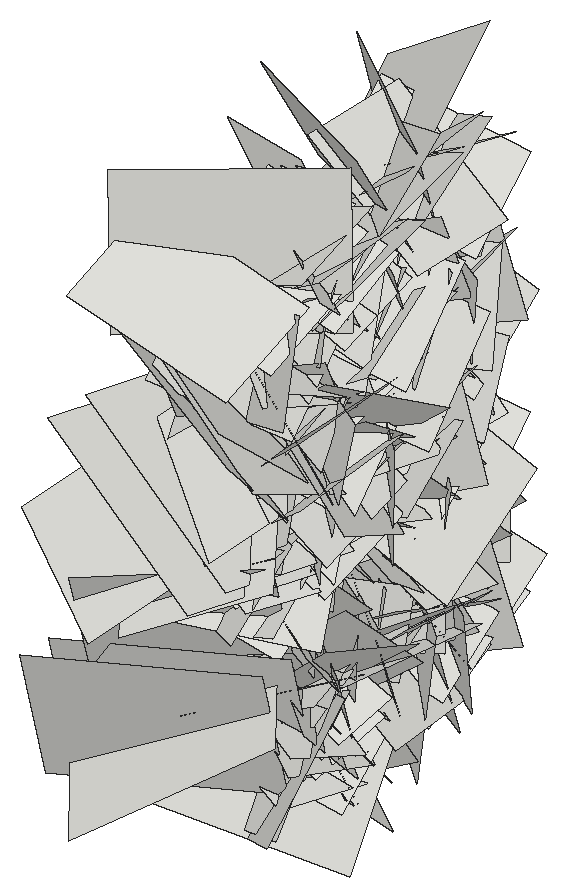
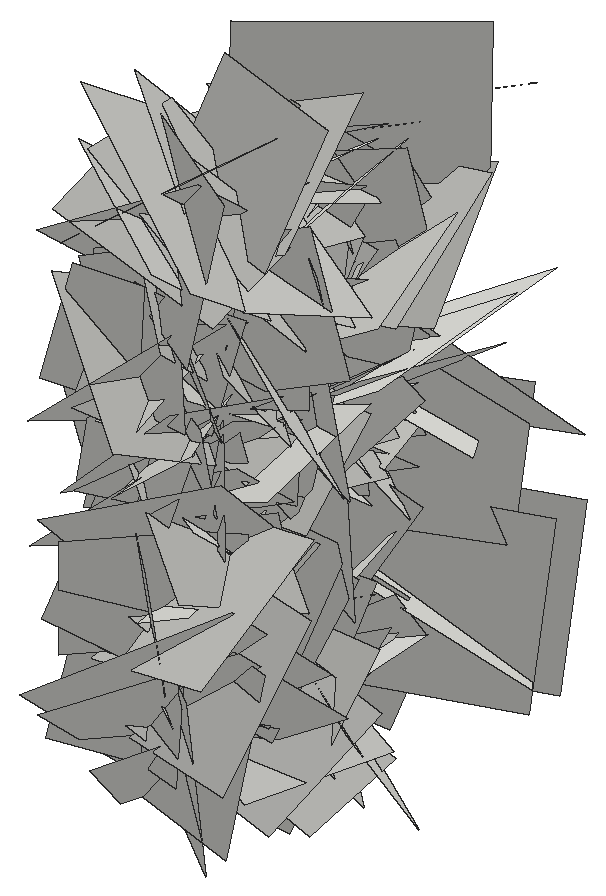
# SketchUp Ruby script. Lengths in inches.
U = 1.inch
M = Sketchup.active_model
def pt(a) = Geom::Point3d.new(a.map { |v| v * U })
def face(e, loops, mat)
  f = e.add_face(loops[0].map { |a| pt(a) })
  loops[1..].each { |l| e.add_face(l.map { |a| pt(a) }).erase! }
  f.material = f.back_material = mat if mat
  f
end
# faces: each face lists its corners as indices into pts; further lists are holes
def faces(e, pts, list, mat = nil) = list.each { |f| face(e, (f[0].is_a?(Array) ? f : [f]).map { |l| l.map { |i| pts[i] } }, mat) }
# xy, xz, yz: faces in a plane at the given z, y or x. An outline is a flat list of corners, or four numbers for a rectangle; further outlines are holes
def ring(l) = l.size == 4 ? [[l[0], l[1]], [l[2], l[1]], [l[2], l[3]], [l[0], l[3]]] : l.each_slice(2).to_a
def flat(e, list, mat, &to3) = list.each { |f| face(e, (f[0].is_a?(Array) ? f : [f]).map { |l| ring(l).map { |u, v| to3.(u, v) } }, mat) }
def xy(e, z, list, mat = nil) = flat(e, list, mat) { |x, y| [x, y, z] }
def xz(e, y, list, mat = nil) = flat(e, list, mat) { |x, z| [x, y, z] }
def yz(e, x, list, mat = nil) = flat(e, list, mat) { |y, z| [x, y, z] }
def lines(e, pts, list) = list.each { |a, b| e.add_line(pt(pts[a]), pt(pts[b])) }
# prism: a flat outline (further loops are holes) pulled along v
def prism(e, loops, v, mat = nil)
  f = face(e, loops, mat); d = Geom::Vector3d.new(v.map { |x| x * U })
  f.pushpull(f.normal.samedirection?(d) ? d.length : -d.length)
end
def box(e, o, s, mat = nil) = prism(e, [[o, [o[0] + s[0], o[1], o[2]], [o[0] + s[0], o[1] + s[1], o[2]], [o[0], o[1] + s[1], o[2]]]], [0, 0, s[2]], mat)
def at(x, y, z, deg = 0) = Geom::Transformation.translation(pt([x, y, z])) * Geom::Transformation.rotation(ORIGIN, Z_AXIS, deg.degrees)
def axes(o, x, y, z) = Geom::Transformation.new([*x, 0, *y, 0, *z, 0, *pt(o).to_a, 1])
def part(name) = M.definitions.add(name)
# library, detail: a bought-in or finely detailed component or shape, given as its bounding box
def library(name, o, s) = part(name).tap { |d| box(d.entities, o, s) }
def detail(e, o, s) = box(e.add_group.entities, o, s)
def put(e, d, t, mat = nil) = e.add_instance(d, t).tap { |i| i.material = mat if mat }
def group(e, t, mat = nil) = e.add_group.tap { |g| g.transformation = t; g.material = mat if mat }.entities
root = M.entities
c1 = part("Component\#6")
p = [[0.01,0,0],[0,3.24,4.54],[4.32,3.24,4.54],[4.33,0,0]]
faces(c1.entities,p,[[0,1,2,3]])
put(root,c1,axes([18.61,125.5,13.2],[-1.07209,0.56535,0.5401],[-0.40295,0.41611,-1.14744],[-0.72423,-1.06841,-0.1611]))
put(root,c1,axes([18.5,125.3125,7.6875],[-0.15543,0.49215,-1.26812],[-0.29157,-1.25984,-0.45713],[-1.41209,0.20597,0.23397]))
put(root,c1,axes([18.5,126.76,7.6875],[-0.15543,0.49215,-1.26812],[-0.29157,-1.25984,-0.45713],[-1.41209,0.20597,0.23397]))
put(root,c1,axes([18.5,135.96,3.29],[-0.1622,-0.76384,1.11136],[-0.23079,1.11781,0.7383],[-1.4107,-0.09505,-0.24857]))
put(root,c1,axes([18.5,130.15,15.41],[-0.24379,0.89731,1.03665],[-0.02149,1.04879,-0.91232],[-1.45316,-0.16605,-0.16042]))
put(root,c1,axes([18.5,136.82,5.83],[-0.1656,-1.02965,0.80161],[-0.14776,0.81588,1.02082],[-1.37528,0.03632,-0.2062]))
put(root,c1,axes([18.5,130.78,10.54],[-0.24762,-1.26357,-0.1726],[0.00687,-0.17664,1.28442],[-1.3518,0.23056,0.03815]))
put(root,c1,axes([19.67,124.5,5.79],[-0.83668,1.07369,0.2523],[-0.21003,0.16716,-1.33127],[-1.15009,-0.81162,0.05958]))
put(root,c1,axes([18.5,138.98,4.78],[-0.22268,-0.9196,-0.8307],[-0.07298,-0.83259,0.9391],[-1.31157,0.20246,0.08879]))
put(root,c1,axes([18.5,129.98,10.23],[-0.10909,-1.3698,0.20566],[0.00727,0.20572,1.37363],[-1.46824,0.1028,-0.00848]))
put(root,c1,axes([18.5,128.0625,10.23],[-0.10909,-1.3698,0.20566],[0.00727,0.20572,1.37363],[-1.46824,0.1028,-0.00848]))
put(root,c1,axes([18.5,135.39,1.18],[-0.01455,-0.40823,1.27358],[-0.1801,1.26386,0.40328],[-1.40617,-0.15765,-0.06483]))
put(root,c1,axes([18.5,137,19.49],[-0.23927,-0.1296,-1.18474],[-0.04055,-1.20439,0.13904],[-1.26266,0.06324,0.22004]))
put(root,c1,axes([18.5,127.67,13.74],[-0.06329,-0.97705,0.81505],[-0.12838,0.8166,0.97005],[-1.34259,-0.03203,-0.13118]))
put(root,c1,axes([18.5,125.99,1.35],[-0.00241,0.79041,1.08039],[-0.06651,1.07914,-0.78963],[-1.41741,-0.05198,0.03522]))
put(root,c1,axes([18.5,132.12,7.08],[0.00585,1.22451,-0.43101],[-0.11167,-0.42917,-1.22063],[-1.3715,0.04016,0.09755]))
put(root,c1,axes([18.5,133.15,22.79],[-0.15509,1.06813,0.73269],[0.10614,0.74447,-1.06531],[-1.36888,-0.06329,-0.16562]))
put(root,c1,axes([18.5,128.24,17.68],[-0.22785,0.52614,1.07761],[0.06777,1.09826,-0.52347],[-1.26934,-0.03581,-0.22138]))
put(root,c1,axes([18.5,133.04,19.75],[-0.14526,-0.49923,0.95494],[-0.24012,0.95446,0.46647],[-1.11669,-0.1403,-0.22453]))
put(root,c1,axes([18.5,139.8125,5.82],[-0.12038,-0.94885,-0.86303],[0.08352,-0.86993,0.94607],[-1.35702,0.03063,0.13479]))
put(root,c1,axes([18.5,131.95,0.87],[-0.07095,-0.70744,0.83659],[-0.30432,0.82019,0.6706],[-1.12076,-0.17792,-0.23504]))
put(root,c1,axes([18.5,125.82,11.42],[-0.20547,0.4933,-0.99975],[-0.03886,-1.01702,-0.49472],[-1.18108,-0.05236,0.1902]))
put(root,c1,axes([18.5,129.66,12.47],[0.1081,-1.2535,0.58167],[0.00417,0.58351,1.25678],[-1.46479,-0.09085,0.0465]))
put(root,c1,axes([18.5,129.48,20.64],[0.14207,1.22324,0.51937],[-0.11373,0.53026,-1.2212],[-1.40407,0.08082,0.15147]))
put(root,c1,axes([18.5,134.94,17.85],[-0.08672,-0.29938,1.1859],[0.04442,1.18717,0.30259],[-1.29573,0.06074,-0.069]))
put(root,c1,axes([18.5,133.96,9.66],[-0.06967,-1.04066,0.34132],[-0.1454,0.34706,1.03175],[-1.15177,0.01914,-0.15089]))
put(root,c1,axes([18.5,126.61,12.8],[0.1414,-0.87971,0.87765],[-0.19082,0.8597,0.88908],[-1.30331,-0.22132,-0.03495]))
put(root,c1,axes([18.5,129.42,5.47],[0.26825,1.30607,0.06413],[-0.25565,0.11082,-1.30519],[-1.36232,0.23638,0.25756]))
put(root,c1,axes([18.5,136.29,19.65],[-0.239,0.33681,-1.04778],[0.13934,-1.05364,-0.36698],[-1.15826,-0.19625,0.17205]))
put(root,c1,axes([18.5,131.16,1.32],[-0.11103,-1.00768,0.14491],[-0.13016,0.15712,1.00381],[-1.07125,0.08535,-0.13699]))
put(root,c1,axes([18.5,129.81,24.32],[0.08615,-0.07511,-1.33483],[0.12267,-1.33188,0.08199],[-1.41184,-0.12031,-0.07433]))
put(root,c1,axes([14.53,129.35,18.22],[-0.07955,-0.40219,0.442],[-0.06566,0.44831,0.39741],[0.63004,-0.00406,0.09723]))
put(root,c1,axes([18.5,130,20.12],[0.02742,-1.01137,-0.35231],[-0.21232,-0.35076,0.99222],[-1.1152,0.04191,-0.19757]))
put(root,c1,axes([18.5,127.69,20.12],[0.02742,-1.01137,-0.35231],[-0.21232,-0.35076,0.99222],[-1.1152,0.04191,-0.19757]))
put(root,c1,axes([14.53,138.1,17.99],[-0.00934,-0.49027,-0.41508],[-0.1892,-0.3969,0.47259],[0.65411,-0.1218,0.13076]))
put(root,c1,axes([18.5,127.92,6.47],[0.03611,0.05394,1.13531],[-0.09971,1.13206,-0.05096],[-1.20066,-0.09239,0.03838]))
put(root,c1,axes([19.22,124.93,11.12],[-0.54058,0.75668,0.32998],[-0.30141,0.20311,-0.90522],[-0.82148,-0.57246,0.11499]))
put(root,c1,axes([18.5,134.14,22.88],[-0.03825,0.99518,-0.25742],[-0.13842,-0.25993,-0.98657],[-1.08078,-0.00193,0.13547]))
put(root,c1,axes([14.53,134.77,2.57],[-0.05447,0.40704,0.46107],[-0.08155,0.45478,-0.41007],[0.64681,0.09162,-0.01288]))
put(root,c1,axes([18.5,131.18,15.16],[-0.15294,-1.16278,0.39158],[0.28955,0.35393,1.15166],[-1.26792,0.22109,0.21577]))
put(root,c1,axes([18.5,131.94,16.85],[0.08825,-0.96476,0.81898],[0.08011,0.82307,0.9619],[-1.33903,-0.01434,0.11152]))
put(root,c1,axes([18.5,128.56,10.3125],[0.23413,0.04823,1.24691],[-0.1221,1.26168,-0.02839],[-1.31707,-0.10839,0.22429]))
put(root,c1,axes([18.5,133.91,11.1875],[0.02059,0.92356,-0.8814],[0.20413,-0.87353,-0.91107],[-1.33776,-0.11908,-0.15259]))
put(root,c1,axes([18.5,130.99,8.6],[-0.04494,-0.64922,0.68663],[-0.20873,0.6783,0.62918],[-0.97967,-0.11474,-0.16555]))
put(root,c1,axes([18.5,129.625,19.87],[0.14331,0.9196,0.97349],[0.15794,0.96203,-0.92947],[-1.41069,0.20113,-0.00516]))
put(root,c1,axes([18.5,137.87,11.82],[-0.23548,-0.98581,-0.19043],[0.17104,-0.22756,0.98976],[-1.05044,0.18394,0.20385]))
put(root,c1,axes([14.53,131.8,8.64],[-0.08497,0.05507,0.67491],[-0.04101,0.67814,-0.05993],[0.71661,0.04534,0.0766]))
put(root,c1,axes([18.5,134.95,12.42],[-0.03363,0.92541,-1.00089],[0.39451,-0.95725,-0.89685],[-1.39004,-0.29406,-0.23032]))
put(root,c1,axes([14.53,131.9,7.66],[-0.03371,0.19161,0.61883],[-0.06203,0.6162,-0.1938],[0.68388,0.06533,0.01292]))
put(root,c1,axes([18.5,131.74,20.5625],[0.11289,-0.41624,-1.03402],[-0.06809,-1.03929,0.41174],[-1.17957,0.02016,-0.12272]))
put(root,c1,axes([18.5,138.97,11.375],[0.02639,-0.72989,-0.72722],[-0.07911,-0.7268,0.72691],[-1.08928,0.0351,-0.07041]))
put(root,c1,axes([18.5,128.87,2.92],[-0.01411,0.95221,-0.19006],[-0.11482,-0.19035,-0.94606],[-1.02282,0.00823,0.10882]))
put(root,c1,axes([14.53,134.26,15.51],[-0.13639,0.72841,-0.25059],[-0.07067,-0.26364,-0.7321],[0.81346,0.09922,-0.10562]))
put(root,c1,axes([18.5,129.68,16.21],[-0.16446,-0.17941,-0.82447],[-0.07006,-0.83314,0.19373],[-0.89165,0.09856,0.13685]))
put(root,c1,axes([14.53,127.28,0.51],[-0.04452,-0.40985,0.5808],[-0.07759,0.58122,0.40485],[0.7495,0.03582,0.07641]))
put(root,c1,axes([18.5,133.2,0.29],[0.16868,0.00753,1.30134],[0.16064,1.302,-0.02607],[-1.37005,0.15359,0.15716]))
put(root,c1,axes([14.53,134.57,7.51],[-0.06425,-0.0713,-0.65597],[0.02618,-0.65852,0.06929],[0.69893,0.01811,-0.0629]))
put(root,c1,axes([18.5,128.52,17.74],[-0.08604,0.43028,-0.81229],[-0.04293,-0.81633,-0.42838],[-0.97342,-0.00203,0.0907]))
put(root,c1,axes([14.53,132.11,13.83],[-0.12823,-0.67114,-0.46171],[-0.10246,-0.45164,0.68184],[0.85739,-0.15435,0.01243]))
put(root,c1,axes([18.5,133.79,15.82],[-0.11741,-0.82822,-0.37202],[-0.00882,-0.37384,0.83474],[-0.96237,0.10447,0.03774]))
put(root,c1,axes([14.53,131.53,3.64],[-0.03356,0.34972,-0.55611],[0.01458,-0.55628,-0.35061],[0.69619,0.02851,-0.01946]))
put(root,c1,axes([14.53,130.57,14.69],[-0.08088,0.56373,-0.36339],[0.06437,-0.35843,-0.56878],[0.70803,0.09698,0.0102]))
put(root,c1,axes([18.5,130.125,12.36],[0.14413,1.23778,0.56401],[0.30073,0.52855,-1.22835],[-1.41013,0.23923,-0.20431]))
put(root,c1,axes([18.5,129.28,18.375],[-0.15104,-0.37703,-0.77667],[0.00911,-0.78776,0.38083],[-0.9151,0.05438,0.13199]))
put(root,c1,axes([18.5,132.6,22.9],[-0.05818,0.99288,0.05669],[0.07779,0.06066,-0.99145],[-1.05129,-0.05046,-0.07649]))
put(root,c1,axes([14.53,133.3125,17.59],[0.01529,0.27468,0.5349],[0.08187,0.52978,-0.27413],[0.6321,-0.07526,0.02257]))
put(root,c1,axes([14.53,129.84,16.13],[0.05288,0.68465,0.04631],[-0.09068,0.05228,-0.68068],[0.72171,-0.04359,-0.08892]))
put(root,c1,axes([18.5,129.45,15.69],[0.00555,0.72683,0.86308],[0.19522,0.85097,-0.71774],[-1.18002,0.1442,-0.11468]))
put(root,c1,axes([14.53,129.41,10.95],[-0.18775,-0.48629,-0.69123],[0.00245,-0.70652,0.49646],[0.89586,-0.09998,-0.14623]))
put(root,c1,axes([14.53,132.63,6.14],[-0.10731,0.87556,-0.00554],[-0.12201,-0.01884,-0.87366],[0.92006,0.09962,-0.1165]))
put(root,c1,axes([18.5,133.96,12.5],[-0.03937,0.24323,0.81298],[-0.12274,0.80469,-0.24604],[-0.89109,-0.12158,-0.00203]))
put(root,c1,axes([18.5,127.6,6.32],[-0.09105,0.77875,-0.27248],[-0.08108,-0.28029,-0.77696],[-0.87078,-0.05533,0.10084]))
put(root,c1,axes([18.5,133.1,9.3125],[0.02086,0.87239,-0.16813],[-0.14049,-0.16341,-0.8634],[-0.93122,0.04419,0.12649]))
put(root,c1,axes([18.5,131.05,1.96],[0.03915,-1.05631,0.36623],[0.17317,0.36759,1.04378],[-1.17236,0.01903,0.16641]))
put(root,c1,axes([14.53,133.88,6.93],[-0.12434,-0.60409,0.41763],[0.12699,0.40152,0.61444],[0.76804,-0.16419,-0.03398]))
put(root,c1,axes([18.5,136.93,7.59],[0.11136,0.24127,-0.97313],[-0.07388,-0.97433,-0.24909],[-1.06018,0.09324,-0.08486]))
put(root,c1,axes([14.53,130.03,2.94],[-0.11679,-0.3481,0.76621],[-0.04914,0.77408,0.34502],[0.89071,-0.00294,0.1195]))
put(root,c1,axes([14.53,129.23,5.41],[-0.17398,-0.60139,0.60701],[0.02487,0.6147,0.61536],[0.9054,-0.13245,0.09973]))
put(root,c1,axes([18.5,132.5,3.06],[0.12033,-0.77552,-0.96336],[0.26418,-0.93322,0.78062],[-1.28404,-0.26468,0.07033]))
put(root,c1,axes([14.53,129.18,10.77],[0.08644,0.04023,-0.60323],[0.06997,-0.60565,-0.03147],[0.63702,0.06107,0.08531]))
put(root,c1,axes([18.5,132.55,10.48],[0.11298,-1.07137,-0.22101],[0.09706,-0.21254,1.07447],[-1.1555,-0.12261,0.06864]))
put(root,c1,axes([14.53,128.34,18.92],[0.04874,0.38349,0.62334],[-0.06251,0.62448,-0.37984],[0.77325,0.02631,-0.07]))
put(root,c1,axes([14.53,129.8,15.91],[0.05085,-0.71724,0.33006],[-0.13843,0.31891,0.71198],[0.82538,0.09767,0.09907]))
put(root,c1,axes([18.5,127.86,19.19],[0.25173,1.01088,0.57921],[0.04385,0.58343,-1.03521],[-1.23418,0.22691,0.08136]))
put(root,c1,axes([18.5,127.34,21.1],[0.03089,0.79811,0.32897],[-0.11706,0.3299,-0.79059],[-0.90753,-0.01539,0.11317]))
put(root,c1,axes([14.53,133.42,16.97],[-0.14677,0.94615,0.46149],[-0.22557,0.4307,-0.94687],[1.09283,0.21597,-0.13346]))
put(root,c1,axes([14.53,133.96,6.46],[-0.0893,0.11056,0.97068],[-0.19494,0.95507,-0.12474],[1.01706,0.19277,0.06132]))
put(root,c1,axes([18.5,136.53,11.26],[0.01536,-0.64622,-0.54667],[-0.11065,-0.54394,0.64022],[-0.89037,0.05645,-0.089]))
put(root,c1,axes([14.53,131.99,-0.9375],[0.0225,-0.54484,0.50649],[-0.02225,0.50605,0.54525],[0.78821,0.02984,0.00093]))
put(root,c1,axes([18.5,127.95,5.4],[-0.05879,0.74539,0.22064],[-0.10629,0.21249,-0.74307],[-0.81711,-0.08127,0.08079]))
put(root,c1,axes([14.53,125.86,8.82],[0.02658,0.53015,0.39509],[0.11889,0.38623,-0.52538],[0.69069,-0.08688,0.07523]))
put(root,c1,axes([14.53,131.86,3.01],[0.01467,-0.55248,-0.51034],[-0.00827,-0.51051,0.55244],[0.7972,0.00487,0.01512]))
put(root,c1,axes([14.53,136.82,15.87],[-0.16772,-0.74319,-0.48228],[0.03783,-0.49486,0.75087],[0.93836,-0.11289,-0.11647]))
put(root,c1,axes([18.5,125.93,11.7],[-0.16945,0.67455,-0.05214],[-0.09647,-0.07453,-0.68517],[-0.71064,-0.15073,0.10544]))
put(root,c1,axes([18.5,127.92,4.7],[-0.092,0.70183,0.2556],[-0.07294,0.24871,-0.70628],[-0.78837,-0.10491,0.03552]))
put(root,c1,axes([18.5,128.53,16.93],[0.30517,1.08519,-0.55956],[0.1011,-0.59314,-1.10124],[-1.29027,0.21019,-0.21864]))
put(root,c1,axes([14.53,137.37,4.77],[-0.01509,-0.67708,-0.46908],[-0.05072,-0.46768,0.67651],[0.87164,-0.03894,0.03124]))
put(root,c1,axes([18.5,133.14,16.06],[0.03738,-0.31853,0.81486],[-0.04959,0.81367,0.32009],[-0.92608,-0.05642,0.01575]))
put(root,c1,axes([18.5,133.58,20.74],[0.06025,0.71815,0.57437],[0.00066,0.57544,-0.71955],[-0.97476,0.04478,0.03501]))
put(root,c1,axes([18.5,131.35,15.19],[-0.02447,0.82058,-0.14823],[-0.01236,-0.14859,-0.82075],[-0.8838,-0.02064,0.01558]))
put(root,c1,axes([14.53,130.01,4.69],[0.05447,0.12092,0.77662],[-0.06993,0.77619,-0.11649],[0.83019,0.05744,-0.06077]))
put(root,c1,axes([18.5,135.14,15.06],[0.15738,0.18416,-1.10832],[0.16264,-1.1108,-0.16402],[-1.17977,-0.12857,-0.17046]))
put(root,c1,axes([18.5,133.07,14.74],[0.12706,0.28525,0.91315],[-0.02767,0.92092,-0.28425],[-1.01369,0.01061,0.12222]))
put(root,c1,axes([18.5,132.96,18.89],[0.10145,-0.91774,-0.17179],[-0.02227,-0.17476,0.92192],[-0.98945,-0.09016,-0.03837]))
put(root,c1,axes([14.53,135.65,2.32],[-0.1935,-1.06071,0.09437],[-0.13048,0.11613,1.0671],[1.12123,-0.16954,0.14047]))
put(root,c1,axes([14.53,136.42,13.64],[0.14309,-0.55174,0.41683],[-0.03038,0.41987,0.56505],[0.73236,0.12522,-0.058]))
put(root,c1,axes([18.5,137.27,19.36],[0.1763,0.15017,-0.9005],[-0.15684,-0.89878,-0.17721],[-0.95491,0.17535,-0.13715]))
put(root,c1,axes([18.5,130.2,1.79],[0.1042,-0.77086,0.73803],[0.17604,0.74317,0.75412],[-1.11745,0.04519,0.18762]))
put(root,c1,axes([18.5,136.01,11.51],[-0.06598,-0.27091,0.62957],[-0.16839,0.62065,0.25136],[-0.70672,-0.12259,-0.11867]))
put(root,c1,axes([14.53,133.51,8.98],[-0.15319,0.47062,-0.90401],[-0.09722,-0.91536,-0.46187],[1.07594,-0.0157,-0.17044]))
put(root,c1,axes([18.5,126.24,11.02],[-0.17433,0.41563,0.4957],[-0.04437,0.50356,-0.43611],[-0.68427,-0.13854,-0.09801]))
put(root,c1,axes([14.53,132.67,11.61],[-0.16439,-1.14375,-0.17253],[-0.24163,-0.14044,1.13591],[1.20204,-0.18465,0.20475]))
put(root,c1,axes([18.5,132.67,11.61],[0.16439,-1.14375,-0.17253],[0.24163,-0.14044,1.13591],[-1.20204,-0.18465,0.20475]))
put(root,c1,axes([14.53,126.24,11.02],[0.17433,0.41563,0.4957],[0.04437,0.50356,-0.43611],[0.68427,-0.13854,-0.09801]))
put(root,c1,axes([18.5,133.51,8.98],[0.15319,0.47062,-0.90401],[0.09722,-0.91536,-0.46187],[-1.07594,-0.0157,-0.17044]))
put(root,c1,axes([14.53,136.01,11.51],[0.06598,-0.27091,0.62957],[0.16839,0.62065,0.25136],[0.70672,-0.12259,-0.11867]))
put(root,c1,axes([14.53,130.2,1.79],[-0.1042,-0.77086,0.73803],[-0.17604,0.74317,0.75412],[1.11745,0.04519,0.18762]))
put(root,c1,axes([14.53,137.27,19.36],[-0.1763,0.15017,-0.9005],[0.15684,-0.89878,-0.17721],[0.95491,0.17535,-0.13715]))
put(root,c1,axes([18.5,136.42,13.64],[-0.14309,-0.55174,0.41683],[0.03038,0.41987,0.56505],[-0.73236,0.12522,-0.058]))
put(root,c1,axes([18.5,135.65,2.32],[0.1935,-1.06071,0.09437],[0.13048,0.11613,1.0671],[-1.12123,-0.16954,0.14047]))
put(root,c1,axes([14.53,132.96,18.89],[-0.10145,-0.91774,-0.17179],[0.02227,-0.17476,0.92192],[0.98945,-0.09016,-0.03837]))
put(root,c1,axes([14.53,133.07,14.74],[-0.12706,0.28525,0.91315],[0.02767,0.92092,-0.28425],[1.01369,0.01061,0.12222]))
put(root,c1,axes([14.53,135.14,15.06],[-0.15738,0.18416,-1.10832],[-0.16264,-1.1108,-0.16402],[1.17977,-0.12857,-0.17046]))
put(root,c1,axes([18.5,130.01,4.69],[-0.05447,0.12092,0.77662],[0.06993,0.77619,-0.11649],[-0.83019,0.05744,-0.06077]))
put(root,c1,axes([14.53,131.35,15.19],[0.02447,0.82058,-0.14823],[0.01236,-0.14859,-0.82075],[0.8838,-0.02064,0.01558]))
put(root,c1,axes([14.53,133.58,20.74],[-0.06025,0.71815,0.57437],[-0.00066,0.57544,-0.71955],[0.97476,0.04478,0.03501]))
put(root,c1,axes([14.53,133.14,16.06],[-0.03738,-0.31853,0.81486],[0.04959,0.81367,0.32009],[0.92608,-0.05642,0.01575]))
put(root,c1,axes([18.5,137.37,4.77],[0.01509,-0.67708,-0.46908],[0.05072,-0.46768,0.67651],[-0.87164,-0.03894,0.03124]))
put(root,c1,axes([14.53,128.53,16.93],[-0.30517,1.08519,-0.55956],[-0.1011,-0.59314,-1.10124],[1.29027,0.21019,-0.21864]))
put(root,c1,axes([14.53,127.92,4.7],[0.092,0.70183,0.2556],[0.07294,0.24871,-0.70628],[0.78837,-0.10491,0.03552]))
put(root,c1,axes([14.53,125.93,11.7],[0.16945,0.67455,-0.05214],[0.09647,-0.07453,-0.68517],[0.71064,-0.15073,0.10544]))
put(root,c1,axes([18.5,136.82,15.87],[0.16772,-0.74319,-0.48228],[-0.03783,-0.49486,0.75087],[-0.93836,-0.11289,-0.11647]))
put(root,c1,axes([18.5,131.86,3.01],[-0.01467,-0.55248,-0.51034],[0.00827,-0.51051,0.55244],[-0.7972,0.00487,0.01512]))
put(root,c1,axes([18.5,125.86,8.82],[-0.02658,0.53015,0.39509],[-0.11889,0.38623,-0.52538],[-0.69069,-0.08688,0.07523]))
put(root,c1,axes([14.53,127.95,5.4],[0.05879,0.74539,0.22064],[0.10629,0.21249,-0.74307],[0.81711,-0.08127,0.08079]))
put(root,c1,axes([18.5,131.99,-0.9375],[-0.0225,-0.54484,0.50649],[0.02225,0.50605,0.54525],[-0.78821,0.02984,0.00093]))
put(root,c1,axes([14.53,136.53,11.26],[-0.01536,-0.64622,-0.54667],[0.11065,-0.54394,0.64022],[0.89037,0.05645,-0.089]))
put(root,c1,axes([18.5,133.96,6.46],[0.0893,0.11056,0.97068],[0.19494,0.95507,-0.12474],[-1.01706,0.19277,0.06132]))
put(root,c1,axes([18.5,133.42,16.97],[0.14677,0.94615,0.46149],[0.22557,0.4307,-0.94687],[-1.09283,0.21597,-0.13346]))
put(root,c1,axes([14.53,127.34,21.1],[-0.03089,0.79811,0.32897],[0.11706,0.3299,-0.79059],[0.90753,-0.01539,0.11317]))
put(root,c1,axes([14.53,127.86,19.19],[-0.25173,1.01088,0.57921],[-0.04385,0.58343,-1.03521],[1.23418,0.22691,0.08136]))
put(root,c1,axes([18.5,129.8,15.91],[-0.05085,-0.71724,0.33006],[0.13843,0.31891,0.71198],[-0.82538,0.09767,0.09907]))
put(root,c1,axes([18.5,128.34,18.92],[-0.04874,0.38349,0.62334],[0.06251,0.62448,-0.37984],[-0.77325,0.02631,-0.07]))
put(root,c1,axes([14.53,132.55,10.48],[-0.11298,-1.07137,-0.22101],[-0.09706,-0.21254,1.07447],[1.1555,-0.12261,0.06864]))
put(root,c1,axes([18.5,129.18,10.77],[-0.08644,0.04023,-0.60323],[-0.06997,-0.60565,-0.03147],[-0.63702,0.06107,0.08531]))
put(root,c1,axes([14.53,132.5,3.06],[-0.12033,-0.77552,-0.96336],[-0.26418,-0.93322,0.78062],[1.28404,-0.26468,0.07033]))
put(root,c1,axes([18.5,129.23,5.41],[0.17398,-0.60139,0.60701],[-0.02487,0.6147,0.61536],[-0.9054,-0.13245,0.09973]))
put(root,c1,axes([18.5,130.03,2.94],[0.11679,-0.3481,0.76621],[0.04914,0.77408,0.34502],[-0.89071,-0.00294,0.1195]))
put(root,c1,axes([14.53,136.93,7.59],[-0.11136,0.24127,-0.97313],[0.07388,-0.97433,-0.24909],[1.06018,0.09324,-0.08486]))
put(root,c1,axes([18.5,133.88,6.93],[0.12434,-0.60409,0.41763],[-0.12699,0.40152,0.61444],[-0.76804,-0.16419,-0.03398]))
put(root,c1,axes([14.53,131.05,1.96],[-0.03915,-1.05631,0.36623],[-0.17317,0.36759,1.04378],[1.17236,0.01903,0.16641]))
put(root,c1,axes([14.53,133.1,9.3125],[-0.02086,0.87239,-0.16813],[0.14049,-0.16341,-0.8634],[0.93122,0.04419,0.12649]))
put(root,c1,axes([14.53,127.6,6.32],[0.09105,0.77875,-0.27248],[0.08108,-0.28029,-0.77696],[0.87078,-0.05533,0.10084]))
put(root,c1,axes([14.53,133.96,12.5],[0.03937,0.24323,0.81298],[0.12274,0.80469,-0.24604],[0.89109,-0.12158,-0.00203]))
put(root,c1,axes([18.5,132.63,6.14],[0.10731,0.87556,-0.00554],[0.12201,-0.01884,-0.87366],[-0.92006,0.09962,-0.1165]))
put(root,c1,axes([18.5,129.41,10.95],[0.18775,-0.48629,-0.69123],[-0.00245,-0.70652,0.49646],[-0.89586,-0.09998,-0.14623]))
put(root,c1,axes([14.53,129.45,15.69],[-0.00555,0.72683,0.86308],[-0.19522,0.85097,-0.71774],[1.18002,0.1442,-0.11468]))
put(root,c1,axes([18.5,129.84,16.13],[-0.05288,0.68465,0.04631],[0.09068,0.05228,-0.68068],[-0.72171,-0.04359,-0.08892]))
put(root,c1,axes([18.5,133.3125,17.59],[-0.01529,0.27468,0.5349],[-0.08187,0.52978,-0.27413],[-0.6321,-0.07526,0.02257]))
put(root,c1,axes([14.53,132.6,22.9],[0.05818,0.99288,0.05669],[-0.07779,0.06066,-0.99145],[1.05129,-0.05046,-0.07649]))
put(root,c1,axes([14.53,129.28,18.375],[0.15104,-0.37703,-0.77667],[-0.00911,-0.78776,0.38083],[0.9151,0.05438,0.13199]))
put(root,c1,axes([14.53,130.125,12.36],[-0.14413,1.23778,0.56401],[-0.30073,0.52855,-1.22835],[1.41013,0.23923,-0.20431]))
put(root,c1,axes([18.5,130.57,14.69],[0.08088,0.56373,-0.36339],[-0.06437,-0.35843,-0.56878],[-0.70803,0.09698,0.0102]))
put(root,c1,axes([18.5,131.53,3.64],[0.03356,0.34972,-0.55611],[-0.01458,-0.55628,-0.35061],[-0.69619,0.02851,-0.01946]))
put(root,c1,axes([14.53,133.79,15.82],[0.11741,-0.82822,-0.37202],[0.00882,-0.37384,0.83474],[0.96237,0.10447,0.03774]))
put(root,c1,axes([18.5,132.11,13.83],[0.12823,-0.67114,-0.46171],[0.10246,-0.45164,0.68184],[-0.85739,-0.15435,0.01243]))
put(root,c1,axes([14.53,128.52,17.74],[0.08604,0.43028,-0.81229],[0.04293,-0.81633,-0.42838],[0.97342,-0.00203,0.0907]))
put(root,c1,axes([18.5,134.57,7.51],[0.06425,-0.0713,-0.65597],[-0.02618,-0.65852,0.06929],[-0.69893,0.01811,-0.0629]))
